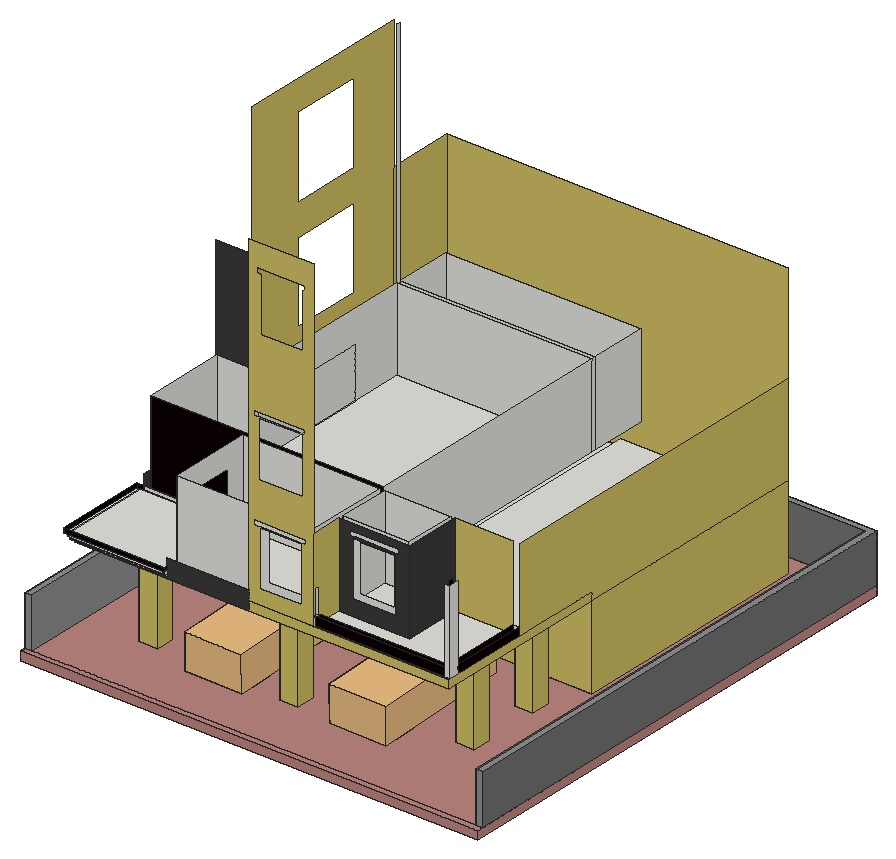
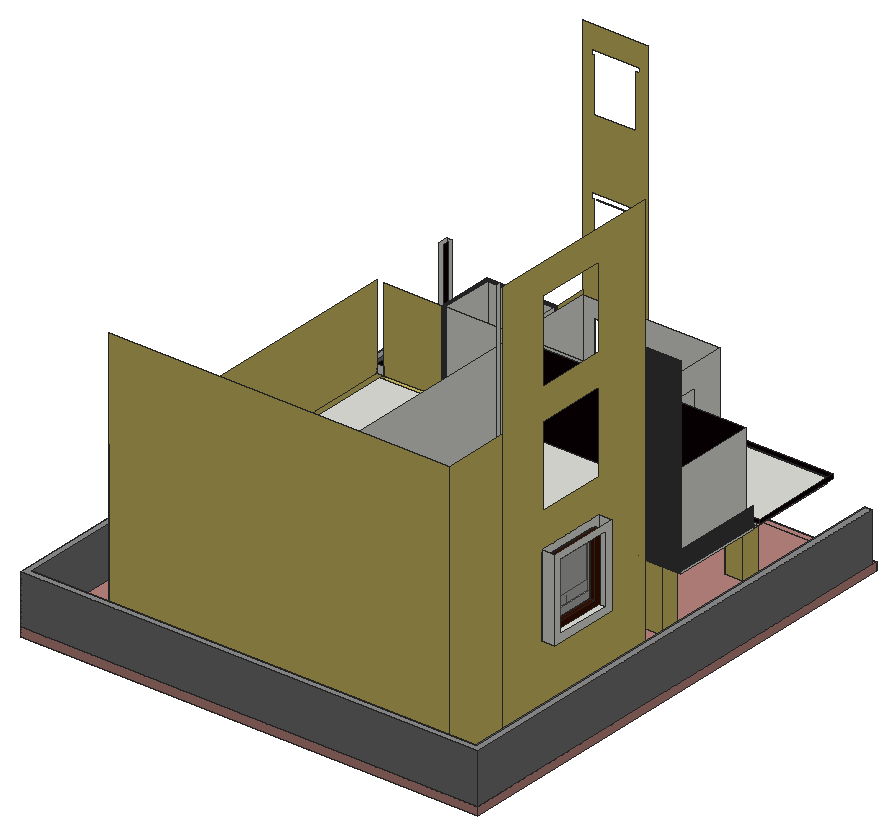
# SketchUp Ruby script. Lengths in inches.
U = 1.inch
M = Sketchup.active_model
def pt(a) = Geom::Point3d.new(a.map { |v| v * U })
def face(e, loops, mat)
  f = e.add_face(loops[0].map { |a| pt(a) })
  loops[1..].each { |l| e.add_face(l.map { |a| pt(a) }).erase! }
  f.material = f.back_material = mat if mat
  f
end
# faces: each face lists its corners as indices into pts; further lists are holes
def faces(e, pts, list, mat = nil) = list.each { |f| face(e, (f[0].is_a?(Array) ? f : [f]).map { |l| l.map { |i| pts[i] } }, mat) }
# xy, xz, yz: faces in a plane at the given z, y or x. An outline is a flat list of corners, or four numbers for a rectangle; further outlines are holes
def ring(l) = l.size == 4 ? [[l[0], l[1]], [l[2], l[1]], [l[2], l[3]], [l[0], l[3]]] : l.each_slice(2).to_a
def flat(e, list, mat, &to3) = list.each { |f| face(e, (f[0].is_a?(Array) ? f : [f]).map { |l| ring(l).map { |u, v| to3.(u, v) } }, mat) }
def xy(e, z, list, mat = nil) = flat(e, list, mat) { |x, y| [x, y, z] }
def xz(e, y, list, mat = nil) = flat(e, list, mat) { |x, z| [x, y, z] }
def yz(e, x, list, mat = nil) = flat(e, list, mat) { |y, z| [x, y, z] }
def lines(e, pts, list) = list.each { |a, b| e.add_line(pt(pts[a]), pt(pts[b])) }
# prism: a flat outline (further loops are holes) pulled along v
def prism(e, loops, v, mat = nil)
  f = face(e, loops, mat); d = Geom::Vector3d.new(v.map { |x| x * U })
  f.pushpull(f.normal.samedirection?(d) ? d.length : -d.length)
end
def box(e, o, s, mat = nil) = prism(e, [[o, [o[0] + s[0], o[1], o[2]], [o[0] + s[0], o[1] + s[1], o[2]], [o[0], o[1] + s[1], o[2]]]], [0, 0, s[2]], mat)
def at(x, y, z, deg = 0) = Geom::Transformation.translation(pt([x, y, z])) * Geom::Transformation.rotation(ORIGIN, Z_AXIS, deg.degrees)
def axes(o, x, y, z) = Geom::Transformation.new([*x, 0, *y, 0, *z, 0, *pt(o).to_a, 1])
def part(name) = M.definitions.add(name)
# library, detail: a bought-in or finely detailed component or shape, given as its bounding box
def library(name, o, s) = part(name).tap { |d| box(d.entities, o, s) }
def detail(e, o, s) = box(e.add_group.entities, o, s)
def put(e, d, t, mat = nil) = e.add_instance(d, t).tap { |i| i.material = mat if mat }
def group(e, t, mat = nil) = e.add_group.tap { |g| g.transformation = t; g.material = mat if mat }.entities
root = M.entities
M.materials.add("[Color C08]").color = [60, 17, 0]
M.materials.add("[Color D05]").color = [208, 191, 99]
M.materials.add("[Color M04]").color = [142, 142, 142]
M.materials.add("[Color M05]").color = [114, 114, 114]
M.materials.add("[Color M07]").color = [58, 58, 58]
M.materials.add("[Concrete Scored Jointless]").color = [188, 133, 127]
M.materials.add("[Metal Seamed]").color = [11, 0, 4]
M.materials.add("[Translucent Glass Gray]").color = [128, 128, 128]
M.materials["[Translucent Glass Gray]"].alpha = 0.5
c1 = library("skp28\#1",[-2.51,-5.3125,0.36],[4.33,10.51,2.73])
c2 = part("ske164\#1")
put(c2.entities,c1,axes([101.27,98.68,1.14],[21.38,0,0],[0,21.38,0],[0,0,21.38]))
c3 = library("ske17D",[0,0,0],[82.9,31.14,82.9])
c4 = part("Sedan car")
put(c4.entities,c2,at(-47.7,14.91,-2.5))
put(c4.entities,c3,axes([87.34,31.1,0],[0,0.35842,0],[-0.35842,0,0],[0,0,0.35842]))
put(c4.entities,c3,axes([87.34,160.85,0],[0,0.35842,0],[-0.35842,0,0],[0,0,0.35842]))
put(c4.entities,c3,axes([5.18,190.5625,0],[0,-0.35842,0],[0.35842,0,0],[0,0,0.35842]))
put(c4.entities,c3,axes([5.43,60.8125,0],[0,-0.35842,0],[0.35842,0,0],[0,0,0.35842]))
c5 = part("Audi car")
put(c5.entities,c4,axes([116.24,65.71,-0.51],[0.88343,0,-0.01128],[0.00041,0.88291,0.03237],[0.01127,-0.03237,0.88283]))
c6 = part("Group\#2")
xy(c6.entities,0,[[0,0,43.625,4]],"[Color C08]")
xy(c6.entities,4.9,[[4.9,0,38.73,4]],"[Color C08]")
xy(c6.entities,53.48,[[4.9,0,38.73,4]],"[Color C08]")
xy(c6.entities,58.375,[[0,0,43.625,4]],"[Color C08]")
xz(c6.entities,0,[[[0,0,43.625,58.375],[4.9,4.9,38.73,53.48]]],"[Color C08]")
xz(c6.entities,0,[[4.9,4.9,38.73,53.48]],"[Translucent Glass Gray]")
xz(c6.entities,4,[[[0,0,43.625,58.375],[4.9,4.9,38.73,53.48]]],"[Color C08]")
yz(c6.entities,0,[[0,0,4,58.375]],"[Color C08]")
yz(c6.entities,4.9,[[0,4.9,4,53.48]],"[Color C08]")
yz(c6.entities,38.73,[[0,4.9,4,53.48]],"[Color C08]")
yz(c6.entities,43.625,[[0,0,4,58.375]],"[Color C08]")
xy(root,0,[[0,0,660,720]],"[Concrete Scored Jointless]")
xy(root,12,[[0,9,0,720,660,720,660,9,651,9,651,711,9,711,9,9],[[72.6875,326.53,564.3125,679.25],[78.6875,332.53,558.3125,624.375]],[78.6875,332.53,558.3125,624.375]])
xy(root,12,[[298.31,95.35,324.93,121.98],[513.65,143.12,540.28,169.74],[513.65,249.68,540.28,276.31],[82.55,256.01,109.17,282.64]],"[Color D05]")
xy(root,12,[[0,0,660,9],[[9,9,651,711],[72.6875,326.53,564.3125,679.25],[298.31,95.35,324.93,121.98],[82.55,256.01,109.17,282.64],[513.65,249.68,540.28,276.31],[513.65,143.12,540.28,169.74],[90.09,101.45,116.72,128.07]]],"[Concrete Scored Jointless]")
xy(root,84,[[0,9,9,9,9,711,651,711,651,9,660,9,660,720,0,720]],"[Color M04]")
xy(root,109.04,[[55.1875,409.31,72.6875,512.1]])
xy(root,119.34,[[55.1875,419.61,72.6875,501.8],[72.6875,419.61,81.6875,501.8]])
xy(root,132,[[78.6875,332.53,558.3125,624.375]])
xy(root,132,[[[24.5,67.28,24.5,195.41,21.75,195.41,21.75,326.53,564.3125,326.53,564.3125,67.28],[82.55,256.01,109.17,282.64],[90.09,101.45,116.72,128.07],[298.31,95.35,324.93,121.98],[513.65,249.68,540.28,276.31],[513.65,143.12,540.28,169.74]]],"[Color D05]")
xy(root,135.375,[[19.625,65.35,19.625,195.41,24.5,195.41,24.5,67.28,21.75,67.28,21.75,65.35],[21.75,65.35,158,67.28],[24.5,67.28,158,195.41]])
xy(root,138.75,[[16.75,63.97,16.75,195.41,19.625,195.41,19.625,65.35,21.75,65.35,21.75,63.97],[19.625,65.35,19.625,195.41,158,195.41,158,66.03,21.75,66.03,21.75,65.35],[21.75,65.35,158,66.03]])
xy(root,138.8125,[[21.75,63.97,158,66.03]])
xy(root,142.375,[[12.3125,62.41,12.3125,195.41,16.75,195.41,16.75,63.97,21.75,63.97,21.75,62.41],[21.75,62.41,158,63.97],[16.75,63.97,158,195.41]])
xy(root,144,[[369.3125,67.28,564.3125,70.41],[369.3125,70.41,369.3125,77.3,556.3,77.3,555.3125,195.41,564.3125,195.41,564.3125,70.41],[165.5625,76.28,363.3125,195.41],[369.3125,77.3,556.3,77.3,555.3125,195.41,471.3125,195.41,471.3125,113.66,369.3125,113.66],[369.3125,119.66,465.3125,195.41],
  [26.75,201.41,363.3125,201.41,363.3125,578.04,81.6875,578.04,81.6875,320.85,26.75,320.85],[369.3125,201.41,555.3125,621.375],[81.6875,578.04,363.3125,582.91],[81.6875,582.91,363.3125,665.75]])
xz(root,0,[[0,0,660,12]],"[Concrete Scored Jointless]")
xz(root,9,[[0,12,9,84],[651,12,660,84]],"[Color M04]")
xz(root,62.41,[[12.3125,142.375,158,148.4375]],"[Metal Seamed]")
xz(root,63.97,[[16.75,138.75,21.75,138.75,21.75,138.8125,158,138.8125,158,142.375,16.75,142.375]])
xz(root,65.35,[[19.625,135.375,158,138.75]])
xz(root,66.03,[[21.75,138.75,158,138.8125]])
xz(root,67.28,[[275.92,132,564.3125,144],[[275.92,144,369.3125,612.8125],[291.14,306.73,291.14,387.29,350.03,387.29,350.03,387.57,290.34,387.57,290.34,387.29,283.95,387.29,283.95,394.6,357.14,394.6,357.14,387.29,353.83,387.29,353.83,306.73],[291.9,166.3,291.9,245.34,349.28,245.34,349.28,245.63,283.19,245.63,283.19,252.66,359.01,252.66,359.01,245.63,353.07,245.63,353.07,166.3],[294.14,495.55,294.14,572.84,287.75,572.84,287.75,580.15,357.625,580.15,357.625,572.84,353.83,572.84,353.83,495.55]]],"[Color D05]")
xz(root,67.28,[[24.5,132,275.92,132,275.92,158.9375,158,158.9375,158,135.375,24.5,135.375]],"[Color M07]")
xz(root,70.41,[[556.3,144,564.3125,144,564.3125,264,556.3,264,556.3,192,556.3125,192,556.3125,188.2,556.3,188.2]])
xz(root,70.41,[[369.3125,144,556.3,156]],"[Metal Seamed]")
xz(root,76.28,[[[165.5625,144,363.3125,264],[297.45,171.85,347.52,239.79]]])
xz(root,77.3,[[369.3125,144,556.3,156]],"[Metal Seamed]")
xz(root,95.35,[[298.31,12,324.93,132]],"[Color D05]")
xz(root,101.45,[[90.09,12,116.72,132]],"[Color D05]")
xz(root,113.66,[[[369.3125,144,471.3125,264],[388.97,165.94,451.12,245.96],[385.19,246.98,385.19,254.29,455.06,254.29,455.06,246.98,451.27,246.98,451.27,247.26,391.58,247.26,391.58,246.98]]],"[Color M07]")
xz(root,119.66,[[[369.3125,144,465.3125,264],[395.02,171.98,445.08,239.92]]])
xz(root,121.98,[[298.31,12,324.93,132]],"[Color D05]")
xz(root,128.07,[[90.09,12,116.72,132]],"[Color D05]")
xz(root,143.12,[[513.65,12,540.28,132]],"[Color D05]")
xz(root,169.74,[[513.65,12,540.28,132]],"[Color D05]")
xz(root,195.41,[[21.75,132,24.5,135.375],[19.625,135.375,21.75,138.75],[21.75,135.375,158,138.75],[16.75,138.75,21.75,142.375],[21.75,138.75,158,142.375],
  [21.75,142.375,158,148.4375],[165.5625,144,363.3125,264],[369.3125,144,465.3125,264],[555.3125,144,564.3125,156]])
xz(root,195.41,[[471.3125,144,555.3125,264]],"[Color D05]")
xz(root,195.41,[[12.3125,142.375,21.75,148.4375]],"[Metal Seamed]")
xz(root,201.41,[[26.75,144,363.3125,264]],"[Metal Seamed]")
xz(root,249.68,[[513.65,12,540.28,132]],"[Color D05]")
xz(root,256.01,[[82.55,12,109.17,132]],"[Color D05]")
xz(root,276.31,[[513.65,12,540.28,132]],"[Color D05]")
xz(root,282.64,[[82.55,12,109.17,132]],"[Color D05]")
xz(root,320.85,[[26.75,144,81.6875,264]])
xz(root,326.53,[[72.6875,12,564.3125,132]],"[Color D05]")
xz(root,326.53,[[21.75,132,72.6875,408]],"[Color M07]")
xz(root,332.53,[[78.6875,12,558.3125,132]])
xz(root,409.31,[[55.1875,109.04,72.6875,227.14]])
xz(root,419.61,[[55.1875,119.34,72.6875,216.84],[72.6875,119.34,81.6875,216.84]])
xz(root,501.8,[[55.1875,119.34,72.6875,216.84],[72.6875,119.34,81.6875,216.84]])
xz(root,512.1,[[55.1875,109.04,72.6875,227.14]])
xz(root,578.04,[[81.6875,144,363.3125,264]])
xz(root,582.91,[[81.6875,144,363.3125,264]])
xz(root,624.375,[[78.6875,12,558.3125,132]])
xz(root,665.75,[[81.6875,144,363.3125,264]])
xz(root,679.25,[[72.6875,12,564.3125,408]],"[Color D05]")
xz(root,711,[[9,12,651,84]],"[Color M05]")
xz(root,720,[[0,12,660,84]],"[Color M05]")
xz(root,720,[[0,0,660,12]],"[Concrete Scored Jointless]")
yz(root,0,[[9,12,720,84]],"[Color M05]")
yz(root,0,[[0,0,720,12]],"[Concrete Scored Jointless]")
yz(root,9,[[9,12,711,84]],"[Color M04]")
yz(root,12.3125,[[62.41,142.375,195.41,148.4375]],"[Metal Seamed]")
yz(root,16.75,[[63.97,138.75,195.41,142.375]])
yz(root,19.625,[[65.35,135.375,195.41,138.75]])
yz(root,21.75,[[195.41,132,326.53,134.4],[63.97,138.75,66.03,138.8125]])
yz(root,21.75,[[195.41,134.4,326.53,162.97]],"[Color M07]")
yz(root,24.5,[[67.28,132,195.41,135.375]])
yz(root,26.75,[[201.41,144,320.85,264]])
yz(root,55.1875,[[[409.31,109.04,512.1,227.14],[419.61,119.34,501.8,216.84]]])
yz(root,72.6875,[[[409.31,109.04,512.1,227.14],[419.61,119.34,501.8,216.84]]])
yz(root,72.6875,[[[326.53,12,582.91,598.25],[409.31,109.04,512.1,227.14],[409.72,437.76,511.69,555.04],[410.35,276.58,511.06,392.6]],[582.91,12,679.25,408]],"[Color D05]")
yz(root,78.6875,[[332.53,12,624.375,132]])
yz(root,81.6875,[[419.61,119.34,501.8,144],[320.85,144,326.53,264],[326.53,144,419.61,144,419.61,216.84,501.8,216.84,501.8,144,578.04,144,578.04,264,326.53,264],[419.61,144,501.8,216.84],[578.04,144,582.91,598.25],
  [582.91,144,665.75,264]])
yz(root,82.55,[[256.01,12,282.64,132]],"[Color D05]")
yz(root,90.09,[[101.45,12,128.07,132]],"[Color D05]")
yz(root,109.17,[[256.01,12,282.64,132]],"[Color D05]")
yz(root,116.72,[[101.45,12,128.07,132]],"[Color D05]")
yz(root,158,[[65.35,135.375,67.28,138.75],[67.28,135.375,195.41,138.75],[66.03,138.75,67.28,138.75,67.28,142.375,63.97,142.375,63.97,138.8125,66.03,138.8125],[67.28,138.75,195.41,142.375],[62.41,142.375,67.28,144],
  [67.28,142.375,195.41,148.4375]])
yz(root,158,[[62.41,144,67.28,148.4375]],"[Metal Seamed]")
yz(root,165.5625,[[[76.28,144,195.41,264],[120.11,148.4375,168.11,232.4375]]])
yz(root,298.31,[[95.35,12,121.98,132]],"[Color D05]")
yz(root,324.93,[[95.35,12,121.98,132]],"[Color D05]")
yz(root,363.3125,[[76.28,144,195.41,264],[201.41,144,578.04,264],[578.04,144,582.91,264],[582.91,144,665.75,264]])
yz(root,369.3125,[[67.28,144,70.41,156],[70.41,144,77.3,156],[119.66,144,195.41,264]])
yz(root,369.3125,[[77.3,144,113.66,144,113.66,264,67.28,264,67.28,156,70.41,156,70.41,192,77.3,192]],"[Color D05]")
yz(root,465.3125,[[119.66,144,195.41,264]])
yz(root,471.3125,[[113.66,144,195.41,264]],"[Color M07]")
yz(root,513.65,[[143.12,12,169.74,132],[249.68,12,276.31,132]],"[Color D05]")
yz(root,540.28,[[143.12,12,169.74,132],[249.68,12,276.31,132]],"[Color D05]")
yz(root,558.3125,[[332.53,12,624.375,132]])
yz(root,564.3125,[[70.41,144,84.63,264]])
yz(root,564.3125,[[326.53,12,679.25,132],[67.28,132,326.53,144],[326.53,132,679.25,132,679.25,264,195.41,264,195.41,144,326.53,144]],"[Color D05]")
yz(root,564.3125,[[84.63,144,195.41,156]],"[Metal Seamed]")
yz(root,651,[[9,12,711,84]],"[Color M05]")
yz(root,660,[[9,12,720,84]],"[Color M05]")
yz(root,660,[[0,0,720,12]],"[Concrete Scored Jointless]")
p = [[555.3125,195.41,144],[556.3,77.3,144],[556.3,77.3,156],[556.3,77.3,188.2],[556.3,77.3,192],[556.3,77.3,264.0625],
  [556.24,84.63,264.0625],[556.24,84.63,192.96],[556.24,84.63,189.95],[556.24,84.63,156],[555.3125,195.41,156],[78.6875,332.53,132],
  [78.6875,332.53,144],[558.3125,332.53,132],[558.3125,332.53,144],[78.6875,461.41,132],[78.6875,461.41,144],[78.6875,495.72,132],
  [78.6875,495.72,144],[555.3125,201.41,144],[363.3125,76.28,144],[363.3125,67.28,144],[81.6875,320.85,144],[81.6875,320.85,134.375],
  [81.6875,338.22,144],[72.6875,338.22,144],[26.75,320.85,144],[26.75,326.53,144],[81.6875,578.04,144],[81.6875,578.04,123]]
faces(root,p,[[0,1,2,3,4,5,6,7,8,9,10]],"[Metal Seamed]")
lines(root,p,[[11,12],[13,14],[15,16],[17,18],[0,19],[20,21],[22,23],[24,25],[26,27],[28,29]])
put(root,c5,at(62.16,9,12))
put(root,c5,at(265.91,14.62,13.55))
put(root,c6,axes([71.14,501.8,119.34],[0,-1.88395,0],[-1.8,0,0],[0,0,1.67024]))
